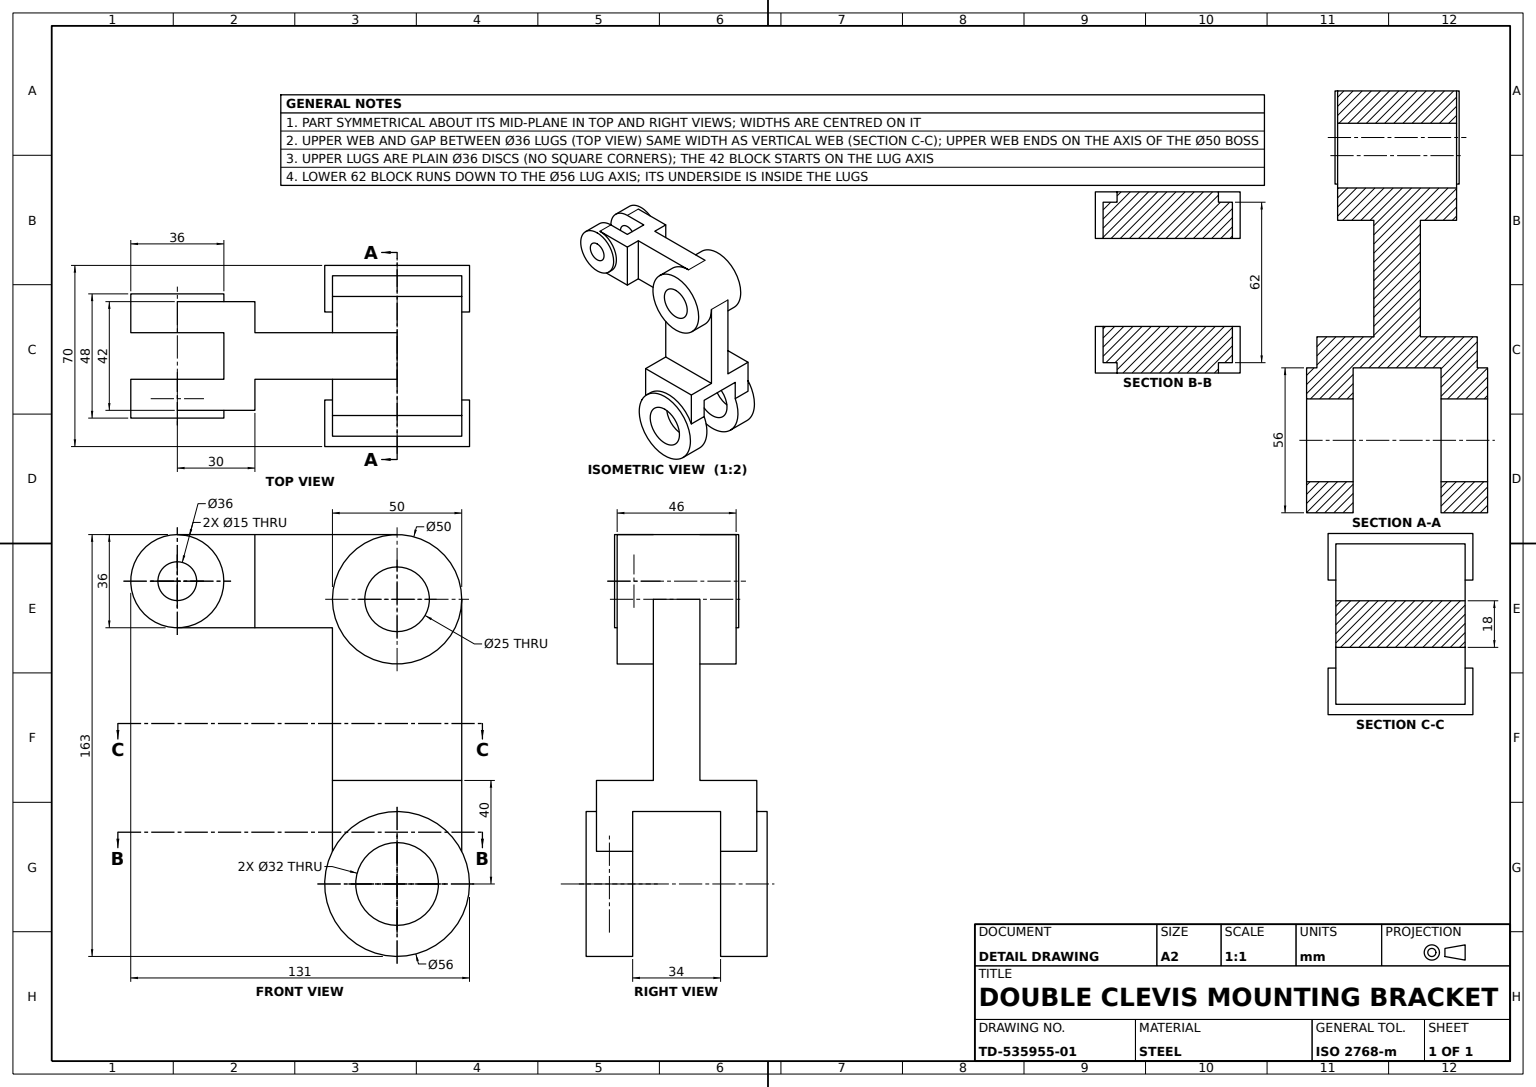
ISO-10303-21;
HEADER;
FILE_DESCRIPTION((''),'2;1');
FILE_NAME('','',(''),(''),'','','');
FILE_SCHEMA(('AUTOMOTIVE_DESIGN'));
ENDSEC;
DATA;
#1=APPLICATION_CONTEXT('');
#2=PRODUCT_CONTEXT('',#1,'mechanical');
#3=PRODUCT('','','',(#2));
#4=PRODUCT_DEFINITION_FORMATION('','',#3);
#5=PRODUCT_DEFINITION_CONTEXT('',#1,'design');
#6=PRODUCT_DEFINITION('','',#4,#5);
#7=PRODUCT_DEFINITION_SHAPE('','',#6);
#8=(LENGTH_UNIT()NAMED_UNIT(*)SI_UNIT(.MILLI.,.METRE.));
#9=(NAMED_UNIT(*)PLANE_ANGLE_UNIT()SI_UNIT($,.RADIAN.));
#10=(NAMED_UNIT(*)SI_UNIT($,.STERADIAN.)SOLID_ANGLE_UNIT());
#11=UNCERTAINTY_MEASURE_WITH_UNIT(LENGTH_MEASURE(0.005),#8,'distance_accuracy_value','');
#12=(GEOMETRIC_REPRESENTATION_CONTEXT(3)GLOBAL_UNCERTAINTY_ASSIGNED_CONTEXT((#11))GLOBAL_UNIT_ASSIGNED_CONTEXT((#8,#9,#10))REPRESENTATION_CONTEXT('',''));
#13=CARTESIAN_POINT('',(23.,0.,122.5));
#14=VERTEX_POINT('',#13);
#15=CARTESIAN_POINT('',(23.,0.,110.));
#16=DIRECTION('',(-1.,0.,0.));
#17=DIRECTION('',(0.,0.,1.));
#18=AXIS2_PLACEMENT_3D('',#15,#16,#17);
#19=CIRCLE('',#18,12.5);
#20=EDGE_CURVE('',#14,#14,#19,.T.);
#21=ORIENTED_EDGE('',*,*,#20,.F.);
#22=EDGE_LOOP('',(#21));
#23=FACE_BOUND('',#22,.T.);
#24=CARTESIAN_POINT('',(-23.,0.,97.5));
#25=VERTEX_POINT('',#24);
#26=CARTESIAN_POINT('',(-23.,0.,110.));
#27=DIRECTION('',(1.,0.,0.));
#28=DIRECTION('',(0.,0.,-1.));
#29=AXIS2_PLACEMENT_3D('',#26,#27,#28);
#30=CIRCLE('',#29,12.5);
#31=EDGE_CURVE('',#25,#25,#30,.T.);
#32=ORIENTED_EDGE('',*,*,#31,.F.);
#33=EDGE_LOOP('',(#32));
#34=FACE_BOUND('',#33,.T.);
#35=CYLINDRICAL_SURFACE('',#18,12.5);
#36=ADVANCED_FACE('',(#23,#34),#35,.F.);
#37=CARTESIAN_POINT('',(9.,-55.,99.));
#38=VERTEX_POINT('',#37);
#39=CARTESIAN_POINT('',(9.,-25.,99.));
#40=VERTEX_POINT('',#39);
#41=CARTESIAN_POINT('',(9.,-85.,99.));
#42=DIRECTION('',(0.,1.,0.));
#43=VECTOR('',#42,1000.);
#44=LINE('',#41,#43);
#45=EDGE_CURVE('',#38,#40,#44,.T.);
#46=ORIENTED_EDGE('',*,*,#45,.T.);
#47=CARTESIAN_POINT('',(9.,-25.,40.));
#48=VERTEX_POINT('',#47);
#49=CARTESIAN_POINT('',(9.,-25.,110.));
#50=VECTOR('',#28,1000.);
#51=LINE('',#49,#50);
#52=EDGE_CURVE('',#40,#48,#51,.T.);
#53=ORIENTED_EDGE('',*,*,#52,.T.);
#54=CARTESIAN_POINT('',(9.,25.,40.));
#55=VERTEX_POINT('',#54);
#56=LINE('',#47,#43);
#57=EDGE_CURVE('',#48,#55,#56,.T.);
#58=ORIENTED_EDGE('',*,*,#57,.T.);
#59=CARTESIAN_POINT('',(9.,25.,110.));
#60=VERTEX_POINT('',#59);
#61=LINE('',#59,#50);
#62=EDGE_CURVE('',#60,#55,#61,.T.);
#63=ORIENTED_EDGE('',*,*,#62,.F.);
#64=CARTESIAN_POINT('',(9.,0.,135.));
#65=VERTEX_POINT('',#64);
#66=CARTESIAN_POINT('',(9.,0.,110.));
#67=AXIS2_PLACEMENT_3D('',#66,#27,#28);
#68=CIRCLE('',#67,25.);
#69=EDGE_CURVE('',#60,#65,#68,.F.);
#70=ORIENTED_EDGE('',*,*,#69,.T.);
#71=CARTESIAN_POINT('',(9.,-55.,135.));
#72=VERTEX_POINT('',#71);
#73=DIRECTION('',(0.,-1.,0.));
#74=VECTOR('',#73,1000.);
#75=LINE('',#64,#74);
#76=EDGE_CURVE('',#65,#72,#75,.T.);
#77=ORIENTED_EDGE('',*,*,#76,.T.);
#78=CARTESIAN_POINT('',(9.,-55.,110.));
#79=LINE('',#78,#50);
#80=EDGE_CURVE('',#72,#38,#79,.T.);
#81=ORIENTED_EDGE('',*,*,#80,.T.);
#82=EDGE_LOOP('',(#46,#53,#58,#63,#70,#77,#81));
#83=FACE_BOUND('',#82,.T.);
#84=AXIS2_PLACEMENT_3D('',#49,#27,#28);
#85=PLANE('',#84);
#86=ADVANCED_FACE('',(#83),#85,.T.);
#87=CARTESIAN_POINT('',(31.,25.,40.));
#88=VERTEX_POINT('',#87);
#89=VECTOR('',#16,1000.);
#90=LINE('',#87,#89);
#91=EDGE_CURVE('',#88,#55,#90,.T.);
#92=ORIENTED_EDGE('',*,*,#91,.T.);
#93=ORIENTED_EDGE('',*,*,#57,.F.);
#94=CARTESIAN_POINT('',(31.,-25.,40.));
#95=VERTEX_POINT('',#94);
#96=LINE('',#94,#89);
#97=EDGE_CURVE('',#95,#48,#96,.T.);
#98=ORIENTED_EDGE('',*,*,#97,.F.);
#99=LINE('',#87,#74);
#100=EDGE_CURVE('',#88,#95,#99,.T.);
#101=ORIENTED_EDGE('',*,*,#100,.F.);
#102=EDGE_LOOP('',(#92,#93,#98,#101));
#103=FACE_BOUND('',#102,.T.);
#104=AXIS2_PLACEMENT_3D('',#87,#17,#27);
#105=PLANE('',#104);
#106=ADVANCED_FACE('',(#103),#105,.T.);
#107=CARTESIAN_POINT('',(35.,28.,0.));
#108=VERTEX_POINT('',#107);
#109=CARTESIAN_POINT('',(35.,0.,0.));
#110=AXIS2_PLACEMENT_3D('',#109,#27,#42);
#111=CIRCLE('',#110,28.);
#112=EDGE_CURVE('',#108,#108,#111,.T.);
#113=ORIENTED_EDGE('',*,*,#112,.T.);
#114=EDGE_LOOP('',(#113));
#115=FACE_BOUND('',#114,.T.);
#116=CARTESIAN_POINT('',(35.,0.,16.));
#117=VERTEX_POINT('',#116);
#118=AXIS2_PLACEMENT_3D('',#109,#16,#17);
#119=CIRCLE('',#118,16.);
#120=EDGE_CURVE('',#117,#117,#119,.T.);
#121=ORIENTED_EDGE('',*,*,#120,.T.);
#122=EDGE_LOOP('',(#121));
#123=FACE_BOUND('',#122,.T.);
#124=AXIS2_PLACEMENT_3D('',#109,#27,#28);
#125=PLANE('',#124);
#126=ADVANCED_FACE('',(#115,#123),#125,.T.);
#127=CARTESIAN_POINT('',(24.,-67.,117.));
#128=VERTEX_POINT('',#127);
#129=CARTESIAN_POINT('',(24.,-85.,117.));
#130=AXIS2_PLACEMENT_3D('',#129,#27,#42);
#131=CIRCLE('',#130,18.);
#132=EDGE_CURVE('',#128,#128,#131,.T.);
#133=ORIENTED_EDGE('',*,*,#132,.T.);
#134=EDGE_LOOP('',(#133));
#135=FACE_BOUND('',#134,.T.);
#136=CARTESIAN_POINT('',(24.,-85.,124.5));
#137=VERTEX_POINT('',#136);
#138=AXIS2_PLACEMENT_3D('',#129,#16,#17);
#139=CIRCLE('',#138,7.5);
#140=EDGE_CURVE('',#137,#137,#139,.T.);
#141=ORIENTED_EDGE('',*,*,#140,.T.);
#142=EDGE_LOOP('',(#141));
#143=FACE_BOUND('',#142,.T.);
#144=AXIS2_PLACEMENT_3D('',#129,#27,#28);
#145=PLANE('',#144);
#146=ADVANCED_FACE('',(#135,#143),#145,.T.);
#147=CARTESIAN_POINT('',(-9.,-67.,99.));
#148=VERTEX_POINT('',#147);
#149=CARTESIAN_POINT('',(-9.,-67.,135.));
#150=VERTEX_POINT('',#149);
#151=CARTESIAN_POINT('',(-9.,-67.,175.));
#152=LINE('',#151,#50);
#153=EDGE_CURVE('',#148,#150,#152,.F.);
#154=ORIENTED_EDGE('',*,*,#153,.T.);
#155=CARTESIAN_POINT('',(-9.,-85.,135.));
#156=VERTEX_POINT('',#155);
#157=CARTESIAN_POINT('',(-9.,0.,135.));
#158=LINE('',#157,#74);
#159=EDGE_CURVE('',#150,#156,#158,.T.);
#160=ORIENTED_EDGE('',*,*,#159,.T.);
#161=CARTESIAN_POINT('',(-9.,-85.,99.));
#162=VERTEX_POINT('',#161);
#163=CARTESIAN_POINT('',(-9.,-85.,117.));
#164=AXIS2_PLACEMENT_3D('',#163,#27,#42);
#165=CIRCLE('',#164,18.);
#166=EDGE_CURVE('',#156,#162,#165,.T.);
#167=ORIENTED_EDGE('',*,*,#166,.T.);
#168=LINE('',#161,#43);
#169=EDGE_CURVE('',#162,#148,#168,.T.);
#170=ORIENTED_EDGE('',*,*,#169,.T.);
#171=EDGE_LOOP('',(#154,#160,#167,#170));
#172=FACE_BOUND('',#171,.T.);
#173=CARTESIAN_POINT('',(-9.,-77.5,117.));
#174=VERTEX_POINT('',#173);
#175=CIRCLE('',#164,7.5);
#176=EDGE_CURVE('',#174,#174,#175,.T.);
#177=ORIENTED_EDGE('',*,*,#176,.F.);
#178=EDGE_LOOP('',(#177));
#179=FACE_BOUND('',#178,.T.);
#180=AXIS2_PLACEMENT_3D('',#151,#27,#42);
#181=PLANE('',#180);
#182=ADVANCED_FACE('',(#172,#179),#181,.T.);
#183=CARTESIAN_POINT('',(-24.,-85.,109.5));
#184=VERTEX_POINT('',#183);
#185=CARTESIAN_POINT('',(-24.,-85.,117.));
#186=AXIS2_PLACEMENT_3D('',#185,#27,#28);
#187=CIRCLE('',#186,7.5);
#188=EDGE_CURVE('',#184,#184,#187,.T.);
#189=ORIENTED_EDGE('',*,*,#188,.F.);
#190=EDGE_LOOP('',(#189));
#191=FACE_BOUND('',#190,.T.);
#192=ORIENTED_EDGE('',*,*,#176,.T.);
#193=EDGE_LOOP('',(#192));
#194=FACE_BOUND('',#193,.T.);
#195=CYLINDRICAL_SURFACE('',#138,7.5);
#196=ADVANCED_FACE('',(#191,#194),#195,.F.);
#197=CARTESIAN_POINT('',(-17.,-25.,12.60952));
#198=VERTEX_POINT('',#197);
#199=CARTESIAN_POINT('',(-31.,-25.,12.60952));
#200=VERTEX_POINT('',#199);
#201=CARTESIAN_POINT('',(35.,-25.,12.60952));
#202=LINE('',#201,#89);
#203=EDGE_CURVE('',#198,#200,#202,.T.);
#204=ORIENTED_EDGE('',*,*,#203,.F.);
#205=CARTESIAN_POINT('',(-17.,-25.,28.));
#206=VERTEX_POINT('',#205);
#207=CARTESIAN_POINT('',(-17.,-25.,0.));
#208=LINE('',#207,#50);
#209=EDGE_CURVE('',#206,#198,#208,.T.);
#210=ORIENTED_EDGE('',*,*,#209,.F.);
#211=CARTESIAN_POINT('',(17.,-25.,28.));
#212=VERTEX_POINT('',#211);
#213=CARTESIAN_POINT('',(0.,-25.,28.));
#214=LINE('',#213,#89);
#215=EDGE_CURVE('',#212,#206,#214,.T.);
#216=ORIENTED_EDGE('',*,*,#215,.F.);
#217=CARTESIAN_POINT('',(17.,-25.,12.60952));
#218=VERTEX_POINT('',#217);
#219=CARTESIAN_POINT('',(17.,-25.,0.));
#220=VECTOR('',#17,1000.);
#221=LINE('',#219,#220);
#222=EDGE_CURVE('',#218,#212,#221,.T.);
#223=ORIENTED_EDGE('',*,*,#222,.F.);
#224=CARTESIAN_POINT('',(31.,-25.,12.60952));
#225=VERTEX_POINT('',#224);
#226=EDGE_CURVE('',#225,#218,#202,.T.);
#227=ORIENTED_EDGE('',*,*,#226,.F.);
#228=CARTESIAN_POINT('',(31.,-25.,0.));
#229=LINE('',#228,#220);
#230=EDGE_CURVE('',#225,#95,#229,.T.);
#231=ORIENTED_EDGE('',*,*,#230,.T.);
#232=ORIENTED_EDGE('',*,*,#97,.T.);
#233=ORIENTED_EDGE('',*,*,#52,.F.);
#234=CARTESIAN_POINT('',(-9.,-25.,99.));
#235=VERTEX_POINT('',#234);
#236=CARTESIAN_POINT('',(0.,-25.,99.));
#237=LINE('',#236,#89);
#238=EDGE_CURVE('',#40,#235,#237,.T.);
#239=ORIENTED_EDGE('',*,*,#238,.T.);
#240=CARTESIAN_POINT('',(-9.,-25.,40.));
#241=VERTEX_POINT('',#240);
#242=LINE('',#240,#220);
#243=EDGE_CURVE('',#241,#235,#242,.T.);
#244=ORIENTED_EDGE('',*,*,#243,.F.);
#245=CARTESIAN_POINT('',(-31.,-25.,40.));
#246=VERTEX_POINT('',#245);
#247=EDGE_CURVE('',#241,#246,#96,.T.);
#248=ORIENTED_EDGE('',*,*,#247,.T.);
#249=LINE('',#245,#50);
#250=EDGE_CURVE('',#246,#200,#249,.T.);
#251=ORIENTED_EDGE('',*,*,#250,.T.);
#252=EDGE_LOOP('',(#204,#210,#216,#223,#227,#231,#232,#233,#239,#244,#248,#251));
#253=FACE_BOUND('',#252,.T.);
#254=CARTESIAN_POINT('',(0.,-25.,0.));
#255=AXIS2_PLACEMENT_3D('',#254,#73,#28);
#256=PLANE('',#255);
#257=ADVANCED_FACE('',(#253),#256,.T.);
#258=CARTESIAN_POINT('',(21.,-55.,135.));
#259=VERTEX_POINT('',#258);
#260=CARTESIAN_POINT('',(21.,-85.,135.));
#261=VERTEX_POINT('',#260);
#262=LINE('',#258,#74);
#263=EDGE_CURVE('',#259,#261,#262,.T.);
#264=ORIENTED_EDGE('',*,*,#263,.T.);
#265=CARTESIAN_POINT('',(21.,-85.,99.));
#266=VERTEX_POINT('',#265);
#267=CARTESIAN_POINT('',(21.,-85.,117.));
#268=AXIS2_PLACEMENT_3D('',#267,#27,#28);
#269=CIRCLE('',#268,18.);
#270=EDGE_CURVE('',#266,#261,#269,.T.);
#271=ORIENTED_EDGE('',*,*,#270,.F.);
#272=CARTESIAN_POINT('',(21.,-55.,99.));
#273=VERTEX_POINT('',#272);
#274=LINE('',#265,#43);
#275=EDGE_CURVE('',#266,#273,#274,.T.);
#276=ORIENTED_EDGE('',*,*,#275,.T.);
#277=LINE('',#272,#220);
#278=EDGE_CURVE('',#273,#259,#277,.T.);
#279=ORIENTED_EDGE('',*,*,#278,.T.);
#280=EDGE_LOOP('',(#264,#271,#276,#279));
#281=FACE_BOUND('',#280,.T.);
#282=CARTESIAN_POINT('',(21.,0.,0.));
#283=AXIS2_PLACEMENT_3D('',#282,#27,#28);
#284=PLANE('',#283);
#285=ADVANCED_FACE('',(#281),#284,.T.);
#286=CARTESIAN_POINT('',(31.,25.,12.60952));
#287=VERTEX_POINT('',#286);
#288=CARTESIAN_POINT('',(31.,0.,0.));
#289=AXIS2_PLACEMENT_3D('',#288,#27,#28);
#290=CIRCLE('',#289,28.);
#291=EDGE_CURVE('',#287,#225,#290,.T.);
#292=ORIENTED_EDGE('',*,*,#291,.F.);
#293=CARTESIAN_POINT('',(31.,25.,0.));
#294=LINE('',#293,#220);
#295=EDGE_CURVE('',#287,#88,#294,.T.);
#296=ORIENTED_EDGE('',*,*,#295,.T.);
#297=ORIENTED_EDGE('',*,*,#100,.T.);
#298=ORIENTED_EDGE('',*,*,#230,.F.);
#299=EDGE_LOOP('',(#292,#296,#297,#298));
#300=FACE_BOUND('',#299,.T.);
#301=AXIS2_PLACEMENT_3D('',#293,#27,#28);
#302=PLANE('',#301);
#303=ADVANCED_FACE('',(#300),#302,.T.);
#304=CARTESIAN_POINT('',(9.,-67.,135.));
#305=VERTEX_POINT('',#304);
#306=LINE('',#304,#89);
#307=EDGE_CURVE('',#305,#150,#306,.T.);
#308=ORIENTED_EDGE('',*,*,#307,.T.);
#309=ORIENTED_EDGE('',*,*,#153,.F.);
#310=CARTESIAN_POINT('',(9.,-67.,99.));
#311=VERTEX_POINT('',#310);
#312=VECTOR('',#27,1000.);
#313=LINE('',#310,#312);
#314=EDGE_CURVE('',#148,#311,#313,.T.);
#315=ORIENTED_EDGE('',*,*,#314,.T.);
#316=CARTESIAN_POINT('',(9.,-67.,175.));
#317=LINE('',#316,#50);
#318=EDGE_CURVE('',#311,#305,#317,.F.);
#319=ORIENTED_EDGE('',*,*,#318,.T.);
#320=EDGE_LOOP('',(#308,#309,#315,#319));
#321=FACE_BOUND('',#320,.T.);
#322=AXIS2_PLACEMENT_3D('',#316,#73,#28);
#323=PLANE('',#322);
#324=ADVANCED_FACE('',(#321),#323,.T.);
#325=ORIENTED_EDGE('',*,*,#112,.F.);
#326=EDGE_LOOP('',(#325));
#327=FACE_BOUND('',#326,.T.);
#328=ORIENTED_EDGE('',*,*,#291,.T.);
#329=ORIENTED_EDGE('',*,*,#226,.T.);
#330=CARTESIAN_POINT('',(17.,25.,12.60952));
#331=VERTEX_POINT('',#330);
#332=CARTESIAN_POINT('',(17.,0.,0.));
#333=AXIS2_PLACEMENT_3D('',#332,#27,#28);
#334=CIRCLE('',#333,28.);
#335=EDGE_CURVE('',#218,#331,#334,.T.);
#336=ORIENTED_EDGE('',*,*,#335,.T.);
#337=CARTESIAN_POINT('',(35.,25.,12.60952));
#338=LINE('',#337,#89);
#339=EDGE_CURVE('',#287,#331,#338,.T.);
#340=ORIENTED_EDGE('',*,*,#339,.F.);
#341=EDGE_LOOP('',(#328,#329,#336,#340));
#342=FACE_BOUND('',#341,.T.);
#343=CYLINDRICAL_SURFACE('',#118,28.);
#344=ADVANCED_FACE('',(#327,#342),#343,.T.);
#345=ORIENTED_EDGE('',*,*,#120,.F.);
#346=EDGE_LOOP('',(#345));
#347=FACE_BOUND('',#346,.T.);
#348=CARTESIAN_POINT('',(17.,0.,-16.));
#349=VERTEX_POINT('',#348);
#350=CIRCLE('',#333,16.);
#351=EDGE_CURVE('',#349,#349,#350,.T.);
#352=ORIENTED_EDGE('',*,*,#351,.F.);
#353=EDGE_LOOP('',(#352));
#354=FACE_BOUND('',#353,.T.);
#355=CYLINDRICAL_SURFACE('',#118,16.);
#356=ADVANCED_FACE('',(#347,#354),#355,.F.);
#357=ORIENTED_EDGE('',*,*,#215,.T.);
#358=CARTESIAN_POINT('',(-17.,25.,28.));
#359=VERTEX_POINT('',#358);
#360=CARTESIAN_POINT('',(-17.,72.,28.));
#361=LINE('',#360,#74);
#362=EDGE_CURVE('',#206,#359,#361,.F.);
#363=ORIENTED_EDGE('',*,*,#362,.T.);
#364=CARTESIAN_POINT('',(17.,25.,28.));
#365=VERTEX_POINT('',#364);
#366=CARTESIAN_POINT('',(0.,25.,28.));
#367=LINE('',#366,#89);
#368=EDGE_CURVE('',#365,#359,#367,.T.);
#369=ORIENTED_EDGE('',*,*,#368,.F.);
#370=CARTESIAN_POINT('',(17.,72.,28.));
#371=LINE('',#370,#74);
#372=EDGE_CURVE('',#212,#365,#371,.F.);
#373=ORIENTED_EDGE('',*,*,#372,.F.);
#374=EDGE_LOOP('',(#357,#363,#369,#373));
#375=FACE_BOUND('',#374,.T.);
#376=AXIS2_PLACEMENT_3D('',#370,#17,#27);
#377=PLANE('',#376);
#378=ADVANCED_FACE('',(#375),#377,.F.);
#379=ORIENTED_EDGE('',*,*,#80,.F.);
#380=LINE('',#258,#89);
#381=EDGE_CURVE('',#259,#72,#380,.T.);
#382=ORIENTED_EDGE('',*,*,#381,.F.);
#383=ORIENTED_EDGE('',*,*,#278,.F.);
#384=LINE('',#272,#89);
#385=EDGE_CURVE('',#273,#38,#384,.T.);
#386=ORIENTED_EDGE('',*,*,#385,.T.);
#387=EDGE_LOOP('',(#379,#382,#383,#386));
#388=FACE_BOUND('',#387,.T.);
#389=AXIS2_PLACEMENT_3D('',#272,#73,#28);
#390=PLANE('',#389);
#391=ADVANCED_FACE('',(#388),#390,.F.);
#392=ORIENTED_EDGE('',*,*,#20,.T.);
#393=EDGE_LOOP('',(#392));
#394=FACE_BOUND('',#393,.T.);
#395=CARTESIAN_POINT('',(23.,25.,110.));
#396=VERTEX_POINT('',#395);
#397=AXIS2_PLACEMENT_3D('',#15,#27,#42);
#398=CIRCLE('',#397,25.);
#399=EDGE_CURVE('',#396,#396,#398,.T.);
#400=ORIENTED_EDGE('',*,*,#399,.T.);
#401=EDGE_LOOP('',(#400));
#402=FACE_BOUND('',#401,.T.);
#403=AXIS2_PLACEMENT_3D('',#15,#27,#28);
#404=PLANE('',#403);
#405=ADVANCED_FACE('',(#394,#402),#404,.T.);
#406=VERTEX_POINT('',#157);
#407=CARTESIAN_POINT('',(-9.,-55.,135.));
#408=VERTEX_POINT('',#407);
#409=EDGE_CURVE('',#406,#408,#158,.T.);
#410=ORIENTED_EDGE('',*,*,#409,.T.);
#411=CARTESIAN_POINT('',(-21.,-55.,135.));
#412=VERTEX_POINT('',#411);
#413=EDGE_CURVE('',#408,#412,#380,.T.);
#414=ORIENTED_EDGE('',*,*,#413,.T.);
#415=CARTESIAN_POINT('',(-21.,-85.,135.));
#416=VERTEX_POINT('',#415);
#417=LINE('',#411,#74);
#418=EDGE_CURVE('',#412,#416,#417,.T.);
#419=ORIENTED_EDGE('',*,*,#418,.T.);
#420=CARTESIAN_POINT('',(9.,-85.,135.));
#421=LINE('',#420,#89);
#422=EDGE_CURVE('',#156,#416,#421,.T.);
#423=ORIENTED_EDGE('',*,*,#422,.F.);
#424=ORIENTED_EDGE('',*,*,#159,.F.);
#425=ORIENTED_EDGE('',*,*,#307,.F.);
#426=VERTEX_POINT('',#420);
#427=LINE('',#64,#43);
#428=EDGE_CURVE('',#426,#305,#427,.T.);
#429=ORIENTED_EDGE('',*,*,#428,.F.);
#430=EDGE_CURVE('',#261,#426,#421,.T.);
#431=ORIENTED_EDGE('',*,*,#430,.F.);
#432=ORIENTED_EDGE('',*,*,#263,.F.);
#433=ORIENTED_EDGE('',*,*,#381,.T.);
#434=ORIENTED_EDGE('',*,*,#76,.F.);
#435=LINE('',#64,#89);
#436=EDGE_CURVE('',#65,#406,#435,.T.);
#437=ORIENTED_EDGE('',*,*,#436,.T.);
#438=EDGE_LOOP('',(#410,#414,#419,#423,#424,#425,#429,#431,#432,#433,#434,#437));
#439=FACE_BOUND('',#438,.T.);
#440=AXIS2_PLACEMENT_3D('',#64,#28,#16);
#441=PLANE('',#440);
#442=ADVANCED_FACE('',(#439),#441,.F.);
#443=CARTESIAN_POINT('',(-35.,0.,-16.));
#444=VERTEX_POINT('',#443);
#445=CARTESIAN_POINT('',(-35.,0.,0.));
#446=AXIS2_PLACEMENT_3D('',#445,#27,#28);
#447=CIRCLE('',#446,16.);
#448=EDGE_CURVE('',#444,#444,#447,.T.);
#449=ORIENTED_EDGE('',*,*,#448,.T.);
#450=EDGE_LOOP('',(#449));
#451=FACE_BOUND('',#450,.T.);
#452=CARTESIAN_POINT('',(-35.,28.,0.));
#453=VERTEX_POINT('',#452);
#454=AXIS2_PLACEMENT_3D('',#445,#27,#42);
#455=CIRCLE('',#454,28.);
#456=EDGE_CURVE('',#453,#453,#455,.T.);
#457=ORIENTED_EDGE('',*,*,#456,.F.);
#458=EDGE_LOOP('',(#457));
#459=FACE_BOUND('',#458,.T.);
#460=PLANE('',#446);
#461=ADVANCED_FACE('',(#451,#459),#460,.F.);
#462=ORIENTED_EDGE('',*,*,#62,.T.);
#463=ORIENTED_EDGE('',*,*,#91,.F.);
#464=ORIENTED_EDGE('',*,*,#295,.F.);
#465=ORIENTED_EDGE('',*,*,#339,.T.);
#466=CARTESIAN_POINT('',(17.,25.,0.));
#467=LINE('',#466,#220);
#468=EDGE_CURVE('',#331,#365,#467,.T.);
#469=ORIENTED_EDGE('',*,*,#468,.T.);
#470=ORIENTED_EDGE('',*,*,#368,.T.);
#471=CARTESIAN_POINT('',(-17.,25.,12.60952));
#472=VERTEX_POINT('',#471);
#473=CARTESIAN_POINT('',(-17.,25.,0.));
#474=LINE('',#473,#50);
#475=EDGE_CURVE('',#359,#472,#474,.T.);
#476=ORIENTED_EDGE('',*,*,#475,.T.);
#477=CARTESIAN_POINT('',(-31.,25.,12.60952));
#478=VERTEX_POINT('',#477);
#479=EDGE_CURVE('',#472,#478,#338,.T.);
#480=ORIENTED_EDGE('',*,*,#479,.T.);
#481=CARTESIAN_POINT('',(-31.,25.,40.));
#482=VERTEX_POINT('',#481);
#483=LINE('',#481,#50);
#484=EDGE_CURVE('',#482,#478,#483,.T.);
#485=ORIENTED_EDGE('',*,*,#484,.F.);
#486=CARTESIAN_POINT('',(-9.,25.,40.));
#487=VERTEX_POINT('',#486);
#488=EDGE_CURVE('',#487,#482,#90,.T.);
#489=ORIENTED_EDGE('',*,*,#488,.F.);
#490=CARTESIAN_POINT('',(-9.,25.,110.));
#491=VERTEX_POINT('',#490);
#492=LINE('',#486,#220);
#493=EDGE_CURVE('',#487,#491,#492,.T.);
#494=ORIENTED_EDGE('',*,*,#493,.T.);
#495=LINE('',#490,#312);
#496=EDGE_CURVE('',#491,#60,#495,.T.);
#497=ORIENTED_EDGE('',*,*,#496,.T.);
#498=EDGE_LOOP('',(#462,#463,#464,#465,#469,#470,#476,#480,#485,#489,#494,#497));
#499=FACE_BOUND('',#498,.T.);
#500=CARTESIAN_POINT('',(0.,25.,0.));
#501=AXIS2_PLACEMENT_3D('',#500,#73,#28);
#502=PLANE('',#501);
#503=ADVANCED_FACE('',(#499),#502,.F.);
#504=CARTESIAN_POINT('',(-21.,-85.,99.));
#505=VERTEX_POINT('',#504);
#506=CARTESIAN_POINT('',(-21.,-85.,117.));
#507=AXIS2_PLACEMENT_3D('',#506,#27,#28);
#508=CIRCLE('',#507,18.);
#509=EDGE_CURVE('',#505,#416,#508,.T.);
#510=ORIENTED_EDGE('',*,*,#509,.F.);
#511=LINE('',#41,#89);
#512=EDGE_CURVE('',#162,#505,#511,.T.);
#513=ORIENTED_EDGE('',*,*,#512,.F.);
#514=ORIENTED_EDGE('',*,*,#166,.F.);
#515=ORIENTED_EDGE('',*,*,#422,.T.);
#516=EDGE_LOOP('',(#510,#513,#514,#515));
#517=FACE_BOUND('',#516,.T.);
#518=CARTESIAN_POINT('',(-24.,-67.,117.));
#519=VERTEX_POINT('',#518);
#520=AXIS2_PLACEMENT_3D('',#185,#27,#42);
#521=CIRCLE('',#520,18.);
#522=EDGE_CURVE('',#519,#519,#521,.T.);
#523=ORIENTED_EDGE('',*,*,#522,.T.);
#524=EDGE_LOOP('',(#523));
#525=FACE_BOUND('',#524,.T.);
#526=CYLINDRICAL_SURFACE('',#138,18.);
#527=ADVANCED_FACE('',(#517,#525),#526,.T.);
#528=CARTESIAN_POINT('',(-17.,0.,16.));
#529=VERTEX_POINT('',#528);
#530=CARTESIAN_POINT('',(-17.,0.,0.));
#531=AXIS2_PLACEMENT_3D('',#530,#16,#17);
#532=CIRCLE('',#531,16.);
#533=EDGE_CURVE('',#529,#529,#532,.T.);
#534=ORIENTED_EDGE('',*,*,#533,.T.);
#535=EDGE_LOOP('',(#534));
#536=FACE_BOUND('',#535,.T.);
#537=CIRCLE('',#531,28.);
#538=EDGE_CURVE('',#472,#198,#537,.T.);
#539=ORIENTED_EDGE('',*,*,#538,.F.);
#540=ORIENTED_EDGE('',*,*,#475,.F.);
#541=ORIENTED_EDGE('',*,*,#362,.F.);
#542=ORIENTED_EDGE('',*,*,#209,.T.);
#543=EDGE_LOOP('',(#539,#540,#541,#542));
#544=FACE_BOUND('',#543,.T.);
#545=AXIS2_PLACEMENT_3D('',#360,#16,#17);
#546=PLANE('',#545);
#547=ADVANCED_FACE('',(#536,#544),#546,.F.);
#548=ORIENTED_EDGE('',*,*,#456,.T.);
#549=EDGE_LOOP('',(#548));
#550=FACE_BOUND('',#549,.T.);
#551=ORIENTED_EDGE('',*,*,#203,.T.);
#552=CARTESIAN_POINT('',(-31.,0.,0.));
#553=AXIS2_PLACEMENT_3D('',#552,#16,#17);
#554=CIRCLE('',#553,28.);
#555=EDGE_CURVE('',#200,#478,#554,.T.);
#556=ORIENTED_EDGE('',*,*,#555,.T.);
#557=ORIENTED_EDGE('',*,*,#479,.F.);
#558=ORIENTED_EDGE('',*,*,#538,.T.);
#559=EDGE_LOOP('',(#551,#556,#557,#558));
#560=FACE_BOUND('',#559,.T.);
#561=ADVANCED_FACE('',(#550,#560),#343,.T.);
#562=ORIENTED_EDGE('',*,*,#385,.F.);
#563=ORIENTED_EDGE('',*,*,#275,.F.);
#564=VERTEX_POINT('',#41);
#565=EDGE_CURVE('',#266,#564,#511,.T.);
#566=ORIENTED_EDGE('',*,*,#565,.T.);
#567=LINE('',#41,#74);
#568=EDGE_CURVE('',#311,#564,#567,.T.);
#569=ORIENTED_EDGE('',*,*,#568,.F.);
#570=ORIENTED_EDGE('',*,*,#314,.F.);
#571=ORIENTED_EDGE('',*,*,#169,.F.);
#572=ORIENTED_EDGE('',*,*,#512,.T.);
#573=CARTESIAN_POINT('',(-21.,-55.,99.));
#574=VERTEX_POINT('',#573);
#575=LINE('',#504,#43);
#576=EDGE_CURVE('',#505,#574,#575,.T.);
#577=ORIENTED_EDGE('',*,*,#576,.T.);
#578=CARTESIAN_POINT('',(-9.,-55.,99.));
#579=VERTEX_POINT('',#578);
#580=EDGE_CURVE('',#579,#574,#384,.T.);
#581=ORIENTED_EDGE('',*,*,#580,.F.);
#582=EDGE_CURVE('',#579,#235,#168,.T.);
#583=ORIENTED_EDGE('',*,*,#582,.T.);
#584=ORIENTED_EDGE('',*,*,#238,.F.);
#585=ORIENTED_EDGE('',*,*,#45,.F.);
#586=EDGE_LOOP('',(#562,#563,#566,#569,#570,#571,#572,#577,#581,#583,#584,#585));
#587=FACE_BOUND('',#586,.T.);
#588=AXIS2_PLACEMENT_3D('',#41,#17,#27);
#589=PLANE('',#588);
#590=ADVANCED_FACE('',(#587),#589,.F.);
#591=ORIENTED_EDGE('',*,*,#247,.F.);
#592=LINE('',#240,#43);
#593=EDGE_CURVE('',#241,#487,#592,.T.);
#594=ORIENTED_EDGE('',*,*,#593,.T.);
#595=ORIENTED_EDGE('',*,*,#488,.T.);
#596=LINE('',#481,#74);
#597=EDGE_CURVE('',#482,#246,#596,.T.);
#598=ORIENTED_EDGE('',*,*,#597,.T.);
#599=EDGE_LOOP('',(#591,#594,#595,#598));
#600=FACE_BOUND('',#599,.T.);
#601=ADVANCED_FACE('',(#600),#105,.T.);
#602=ORIENTED_EDGE('',*,*,#335,.F.);
#603=ORIENTED_EDGE('',*,*,#222,.T.);
#604=ORIENTED_EDGE('',*,*,#372,.T.);
#605=ORIENTED_EDGE('',*,*,#468,.F.);
#606=EDGE_LOOP('',(#602,#603,#604,#605));
#607=FACE_BOUND('',#606,.T.);
#608=ORIENTED_EDGE('',*,*,#351,.T.);
#609=EDGE_LOOP('',(#608));
#610=FACE_BOUND('',#609,.T.);
#611=CARTESIAN_POINT('',(17.,72.,-34.66957));
#612=AXIS2_PLACEMENT_3D('',#611,#27,#28);
#613=PLANE('',#612);
#614=ADVANCED_FACE('',(#607,#610),#613,.F.);
#615=ORIENTED_EDGE('',*,*,#413,.F.);
#616=CARTESIAN_POINT('',(-9.,-55.,40.));
#617=LINE('',#616,#220);
#618=EDGE_CURVE('',#579,#408,#617,.T.);
#619=ORIENTED_EDGE('',*,*,#618,.F.);
#620=ORIENTED_EDGE('',*,*,#580,.T.);
#621=LINE('',#573,#220);
#622=EDGE_CURVE('',#574,#412,#621,.T.);
#623=ORIENTED_EDGE('',*,*,#622,.T.);
#624=EDGE_LOOP('',(#615,#619,#620,#623));
#625=FACE_BOUND('',#624,.T.);
#626=ADVANCED_FACE('',(#625),#390,.F.);
#627=ORIENTED_EDGE('',*,*,#576,.F.);
#628=ORIENTED_EDGE('',*,*,#509,.T.);
#629=ORIENTED_EDGE('',*,*,#418,.F.);
#630=ORIENTED_EDGE('',*,*,#622,.F.);
#631=EDGE_LOOP('',(#627,#628,#629,#630));
#632=FACE_BOUND('',#631,.T.);
#633=CARTESIAN_POINT('',(-21.,0.,0.));
#634=AXIS2_PLACEMENT_3D('',#633,#27,#28);
#635=PLANE('',#634);
#636=ADVANCED_FACE('',(#632),#635,.F.);
#637=ORIENTED_EDGE('',*,*,#140,.F.);
#638=EDGE_LOOP('',(#637));
#639=FACE_BOUND('',#638,.T.);
#640=CARTESIAN_POINT('',(9.,-92.5,117.));
#641=VERTEX_POINT('',#640);
#642=CARTESIAN_POINT('',(9.,-85.,117.));
#643=AXIS2_PLACEMENT_3D('',#642,#16,#73);
#644=CIRCLE('',#643,7.5);
#645=EDGE_CURVE('',#641,#641,#644,.T.);
#646=ORIENTED_EDGE('',*,*,#645,.T.);
#647=EDGE_LOOP('',(#646));
#648=FACE_BOUND('',#647,.T.);
#649=ADVANCED_FACE('',(#639,#648),#195,.F.);
#650=ORIENTED_EDGE('',*,*,#448,.F.);
#651=EDGE_LOOP('',(#650));
#652=FACE_BOUND('',#651,.T.);
#653=ORIENTED_EDGE('',*,*,#533,.F.);
#654=EDGE_LOOP('',(#653));
#655=FACE_BOUND('',#654,.T.);
#656=ADVANCED_FACE('',(#652,#655),#355,.F.);
#657=ORIENTED_EDGE('',*,*,#597,.F.);
#658=ORIENTED_EDGE('',*,*,#484,.T.);
#659=ORIENTED_EDGE('',*,*,#555,.F.);
#660=ORIENTED_EDGE('',*,*,#250,.F.);
#661=EDGE_LOOP('',(#657,#658,#659,#660));
#662=FACE_BOUND('',#661,.T.);
#663=AXIS2_PLACEMENT_3D('',#481,#16,#17);
#664=PLANE('',#663);
#665=ADVANCED_FACE('',(#662),#664,.T.);
#666=ORIENTED_EDGE('',*,*,#132,.F.);
#667=EDGE_LOOP('',(#666));
#668=FACE_BOUND('',#667,.T.);
#669=ORIENTED_EDGE('',*,*,#430,.T.);
#670=CIRCLE('',#643,18.);
#671=EDGE_CURVE('',#564,#426,#670,.T.);
#672=ORIENTED_EDGE('',*,*,#671,.F.);
#673=ORIENTED_EDGE('',*,*,#565,.F.);
#674=ORIENTED_EDGE('',*,*,#270,.T.);
#675=EDGE_LOOP('',(#669,#672,#673,#674));
#676=FACE_BOUND('',#675,.T.);
#677=ADVANCED_FACE('',(#668,#676),#526,.T.);
#678=ORIENTED_EDGE('',*,*,#409,.F.);
#679=CARTESIAN_POINT('',(-9.,0.,110.));
#680=AXIS2_PLACEMENT_3D('',#679,#16,#17);
#681=CIRCLE('',#680,25.);
#682=EDGE_CURVE('',#406,#491,#681,.F.);
#683=ORIENTED_EDGE('',*,*,#682,.T.);
#684=ORIENTED_EDGE('',*,*,#493,.F.);
#685=ORIENTED_EDGE('',*,*,#593,.F.);
#686=ORIENTED_EDGE('',*,*,#243,.T.);
#687=ORIENTED_EDGE('',*,*,#582,.F.);
#688=ORIENTED_EDGE('',*,*,#618,.T.);
#689=EDGE_LOOP('',(#678,#683,#684,#685,#686,#687,#688));
#690=FACE_BOUND('',#689,.T.);
#691=AXIS2_PLACEMENT_3D('',#240,#16,#17);
#692=PLANE('',#691);
#693=ADVANCED_FACE('',(#690),#692,.T.);
#694=ORIENTED_EDGE('',*,*,#399,.F.);
#695=EDGE_LOOP('',(#694));
#696=FACE_BOUND('',#695,.T.);
#697=ORIENTED_EDGE('',*,*,#69,.F.);
#698=ORIENTED_EDGE('',*,*,#496,.F.);
#699=ORIENTED_EDGE('',*,*,#682,.F.);
#700=ORIENTED_EDGE('',*,*,#436,.F.);
#701=EDGE_LOOP('',(#697,#698,#699,#700));
#702=FACE_BOUND('',#701,.T.);
#703=CARTESIAN_POINT('',(-23.,25.,110.));
#704=VERTEX_POINT('',#703);
#705=AXIS2_PLACEMENT_3D('',#26,#27,#42);
#706=CIRCLE('',#705,25.);
#707=EDGE_CURVE('',#704,#704,#706,.T.);
#708=ORIENTED_EDGE('',*,*,#707,.T.);
#709=EDGE_LOOP('',(#708));
#710=FACE_BOUND('',#709,.T.);
#711=CYLINDRICAL_SURFACE('',#18,25.);
#712=ADVANCED_FACE('',(#696,#702,#710),#711,.T.);
#713=ORIENTED_EDGE('',*,*,#188,.T.);
#714=EDGE_LOOP('',(#713));
#715=FACE_BOUND('',#714,.T.);
#716=ORIENTED_EDGE('',*,*,#522,.F.);
#717=EDGE_LOOP('',(#716));
#718=FACE_BOUND('',#717,.T.);
#719=PLANE('',#186);
#720=ADVANCED_FACE('',(#715,#718),#719,.F.);
#721=ORIENTED_EDGE('',*,*,#428,.T.);
#722=ORIENTED_EDGE('',*,*,#318,.F.);
#723=ORIENTED_EDGE('',*,*,#568,.T.);
#724=ORIENTED_EDGE('',*,*,#671,.T.);
#725=EDGE_LOOP('',(#721,#722,#723,#724));
#726=FACE_BOUND('',#725,.T.);
#727=ORIENTED_EDGE('',*,*,#645,.F.);
#728=EDGE_LOOP('',(#727));
#729=FACE_BOUND('',#728,.T.);
#730=CARTESIAN_POINT('',(9.,-116.,175.));
#731=AXIS2_PLACEMENT_3D('',#730,#16,#73);
#732=PLANE('',#731);
#733=ADVANCED_FACE('',(#726,#729),#732,.T.);
#734=ORIENTED_EDGE('',*,*,#707,.F.);
#735=EDGE_LOOP('',(#734));
#736=FACE_BOUND('',#735,.T.);
#737=ORIENTED_EDGE('',*,*,#31,.T.);
#738=EDGE_LOOP('',(#737));
#739=FACE_BOUND('',#738,.T.);
#740=PLANE('',#29);
#741=ADVANCED_FACE('',(#736,#739),#740,.F.);
#742=CLOSED_SHELL('',(#36,#86,#106,#126,#146,#182,#196,#257,#285,#303,#324,#344,#356,#378,#391,#405,#442,#461,#503,#527,#547,#561,#590,#601,#614,#626,#636,#649,#656,#665,#677,#693,#712,#720,#733,#741));
#743=MANIFOLD_SOLID_BREP('',#742);
#744=ADVANCED_BREP_SHAPE_REPRESENTATION('',(#743),#12);
#745=SHAPE_DEFINITION_REPRESENTATION(#7,#744);
ENDSEC;
END-ISO-10303-21;
